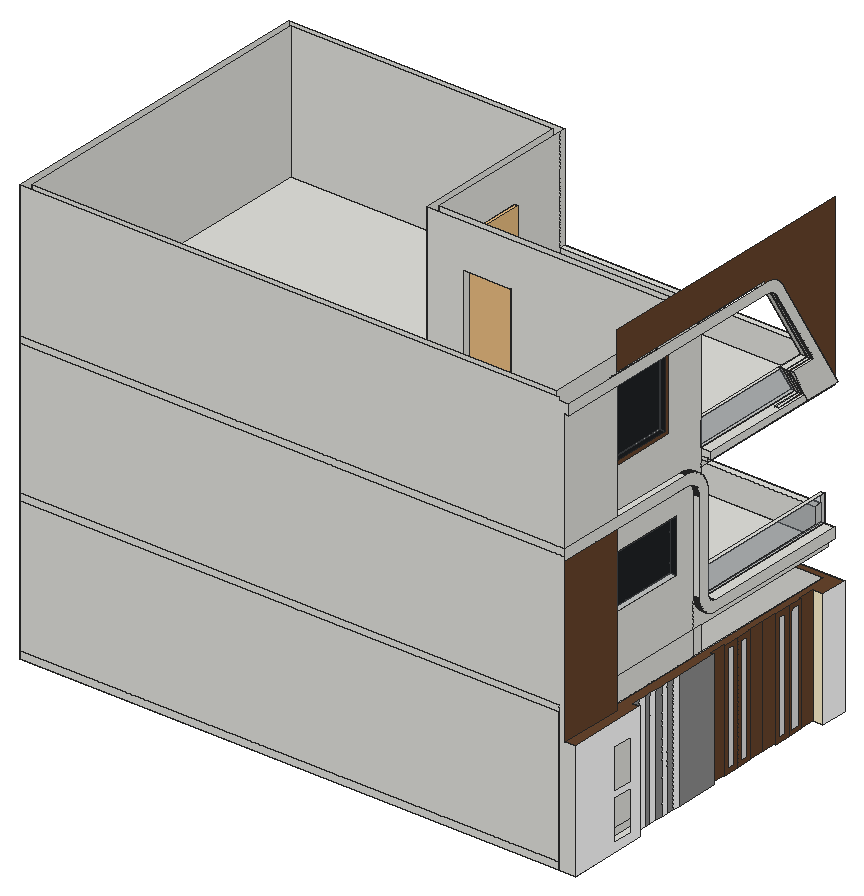
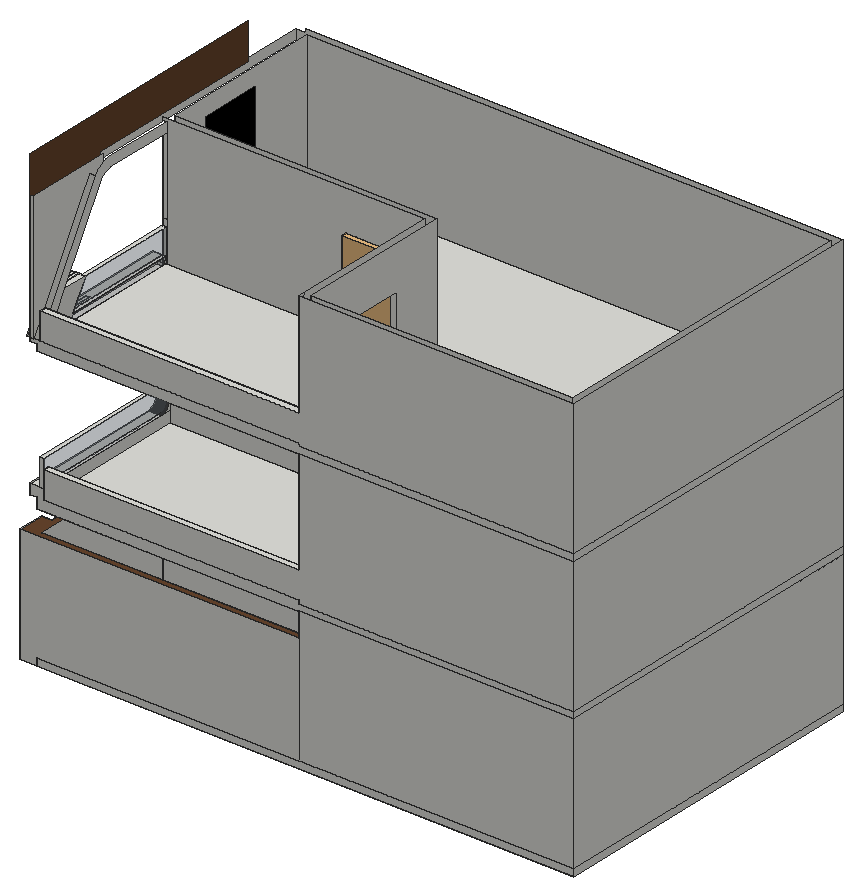
# SketchUp Ruby script. Lengths in inches.
U = 1.inch
M = Sketchup.active_model
def pt(a) = Geom::Point3d.new(a.map { |v| v * U })
def face(e, loops, mat)
  f = e.add_face(loops[0].map { |a| pt(a) })
  loops[1..].each { |l| e.add_face(l.map { |a| pt(a) }).erase! }
  f.material = f.back_material = mat if mat
  f
end
# faces: each face lists its corners as indices into pts; further lists are holes
def faces(e, pts, list, mat = nil) = list.each { |f| face(e, (f[0].is_a?(Array) ? f : [f]).map { |l| l.map { |i| pts[i] } }, mat) }
# xy, xz, yz: faces in a plane at the given z, y or x. An outline is a flat list of corners, or four numbers for a rectangle; further outlines are holes
def ring(l) = l.size == 4 ? [[l[0], l[1]], [l[2], l[1]], [l[2], l[3]], [l[0], l[3]]] : l.each_slice(2).to_a
def flat(e, list, mat, &to3) = list.each { |f| face(e, (f[0].is_a?(Array) ? f : [f]).map { |l| ring(l).map { |u, v| to3.(u, v) } }, mat) }
def xy(e, z, list, mat = nil) = flat(e, list, mat) { |x, y| [x, y, z] }
def xz(e, y, list, mat = nil) = flat(e, list, mat) { |x, z| [x, y, z] }
def yz(e, x, list, mat = nil) = flat(e, list, mat) { |y, z| [x, y, z] }
def lines(e, pts, list) = list.each { |a, b| e.add_line(pt(pts[a]), pt(pts[b])) }
# prism: a flat outline (further loops are holes) pulled along v
def prism(e, loops, v, mat = nil)
  f = face(e, loops, mat); d = Geom::Vector3d.new(v.map { |x| x * U })
  f.pushpull(f.normal.samedirection?(d) ? d.length : -d.length)
end
def box(e, o, s, mat = nil) = prism(e, [[o, [o[0] + s[0], o[1], o[2]], [o[0] + s[0], o[1] + s[1], o[2]], [o[0], o[1] + s[1], o[2]]]], [0, 0, s[2]], mat)
def at(x, y, z, deg = 0) = Geom::Transformation.translation(pt([x, y, z])) * Geom::Transformation.rotation(ORIGIN, Z_AXIS, deg.degrees)
def axes(o, x, y, z) = Geom::Transformation.new([*x, 0, *y, 0, *z, 0, *pt(o).to_a, 1])
def part(name) = M.definitions.add(name)
# library, detail: a bought-in or finely detailed component or shape, given as its bounding box
def library(name, o, s) = part(name).tap { |d| box(d.entities, o, s) }
def detail(e, o, s) = box(e.add_group.entities, o, s)
def put(e, d, t, mat = nil) = e.add_instance(d, t).tap { |i| i.material = mat if mat }
def group(e, t, mat = nil) = e.add_group.tap { |g| g.transformation = t; g.material = mat if mat }.entities
root = M.entities
M.materials.add("D01_Frost_White").color = [255, 242, 206]
M.materials.add("Glass_Basic_01").color = [130, 139, 150]
M.materials["Glass_Basic_01"].alpha = 0.25
M.materials.add("M00_Soft_Cloud").color = [255, 255, 255]
M.materials.add("M01_Silver_Fog").color = [224, 224, 224]
M.materials.add("M04_Stone_Frost").color = [142, 142, 142]
M.materials.add("M09_Shadow_Night").color = [0, 0, 0]
M.materials.add("Wood_Veneer_15_1K").color = [103, 69, 45]
c1 = library("porta+4",[0.2,-5.42,1.33],[46.55,4.72,83.21])
c2 = library("mesh-166",[-1553.69,-2604.3125,-42.18],[1702.88,1401.6,88.28])
c3 = part("Group17")
put(c3.entities,c2,at(294.66,859.51,3.5))
xy(root,-6,[[0,0,480,300],[480,0,480,300,495,300,495,276,486,276,486,261.75,487,261.75,487,233.25,486,233.25,486,204.75,487,204.75,487,176.25,486,176.25,486,162,489,162,489,72,495,72,495,0]])
xy(root,0,[[9,9,369,153],[375,9,471,153],[9,159,240,291],[246,159,471,291],[471,159,480,159,480,294,246,294,246,291,471,291],
  [246,294,480,300]])
xy(root,3,[[273,153,315,159]])
xy(root,39,[[240,198,246,240]])
xy(root,81,[[273,153,315,159],[240,198,246,240]])
xy(root,98.18,[[486,0,495,0,495,72,489,72,489,162,486,162,486,176.25,487,176.25,487,204.75,486,204.75,486,233.25,487,233.25,487,261.75,486,261.75,486,276,495,276,495,300,246,300,246,294,480,294,480,57,486,57]],"Wood_Veneer_15_1K")
xy(root,120,[[0,0,480,0,480,159,471,159,471,9,0,9],[0,9,9,300],[9,9,369,153],[369,9,375,159],[375,9,471,153],
  [9,153,369,153,369,159,246,159,246,300,240,300,240,159,9,159],[375,153,471,159],[9,159,240,291],[246,159,480,291],[9,291,240,300],
  [246,291,480,300]])
xy(root,126,[[6,6,474,6,474,153,240,153,240,294,6,294]])
xy(root,129,[[273,153,315,159],[246,159,474,294],[480,168,486,300],[246,294,474,300]])
xy(root,138,[[474,159,477,168],[474,168,477,300],[477,168,486,300]])
xy(root,153,[[246,294,474,300]])
xy(root,162,[[474,159,477,300]])
xy(root,165,[[240,198,246,240]])
xy(root,171,[[474,60,480,132]])
xy(root,207,[[273,153,315,159],[240,198,246,240]])
xy(root,219,[[474,60,480,108],[474,108,480,132]])
xy(root,243,[[480,57,486,135]])
xy(root,246,[[0,6,6,300],[6,6,6,294,240,294,240,153,474,153,474,6],[240,153,474,153,474,159,246,159,246,300,240,300],[246,159,480,300],[6,294,240,300]])
xy(root,252,[[6,6,474,6,474,153,240,153,240,294,6,294],[480,57,486,135],[480,159,486,300]])
xy(root,255,[[273,153,315,159],[246,159,477,294],[486,159,489,269.77],[483,237.63,486,269.77],[477,269.77,483,291],
  [483,269.77,486,291],[486,269.77,489,291],[477,291,483,300],[483,291,486,300],[486,291,489,300]])
xy(root,261,[[477,159,480,263.46],[480,159,489,159,489,263.46,486,263.46,486,237.63,483,237.63,483,263.46,480,263.46],[483,237.63,486,263.46]])
xy(root,279,[[246,294,477,300]])
xy(root,285,[[477,159,480,249.31],[477,249.31,483,273.31],[483,249.31,486,273.31],[486,249.31,489,273.31]])
xy(root,291,[[240,198,246,240]])
xy(root,291,[[474,63,480,120]],"M09_Shadow_Night")
xy(root,333,[[273,153,315,159],[240,198,246,240]])
xz(root,0,[[0,-6,480,0],[480,-6,495,-6,495,98.18,486,98.18,486,246,0,246,0,126,480,126],[0,0,480,120],[0,120,480,126],[0,246,486,252],
  [0,252,486,252,486,360,489,360,489,368.99,486,368.99,486,369,480,369,480,372,0,372]])
xz(root,6,[[6,126,474,246],[6,252,474,372]])
xz(root,9,[[9,0,369,120],[375,0,471,120]])
xz(root,57,[[480,98.18,486,243],[480,252,486,360]])
xz(root,60,[[474,171,480,219]])
xz(root,63,[[474,291,480,357]],"M09_Shadow_Night")
xz(root,72,[[489,-6,495,98.18]],"Wood_Veneer_15_1K")
xz(root,120,[[474,291,480,357]],"M09_Shadow_Night")
xz(root,132,[[474,171,480,219]],"M09_Shadow_Night")
xz(root,150,[[480,147,486,228]])
xz(root,153,[[[9,0,369,120],[273,3,315,81]],[375,0,471,120],[[240,126,474,246],[273,129,315,207]],[[240,252,474,372],[273,255,315,333]]])
xz(root,159,[[9,0,240,120],[246,0,246,120,480,120,480,0,318,0,318,84,270,84,270,0],[[270,0,318,84],[273,3,315,81]],[246,126,270,129],[270,126,318,129],
  [246,129,246,246,480,246,480,228,486,228,486,147,477,147,477,162,474,162,474,129,318,129,318,210,270,210,270,129],[270,129,270,210,318,210,318,129,315,129,315,207,273,207,273,129],[474,138,477,147],[474,147,477,162],[480,252,486,255],
  [246,255,246,372,480,372,480,369,477,369,477,255,318,255,318,336,270,336,270,255],[270,255,270,336,318,336,318,255,315,255,315,333,273,333,273,255],[477,255,480,261],[480,255,489,261],[477,261,480,285],
  [477,285,480,291],[477,291,480,360]])
xz(root,162,[[486,-6,489,98.18]],"Wood_Veneer_15_1K")
xz(root,176.25,[[486,-6,487,98.18]],"Wood_Veneer_15_1K")
xz(root,198,[[240,39,246,81],[240,165,246,207],[240,291,246,333]])
xz(root,204.75,[[486,-6,487,98.18]],"Wood_Veneer_15_1K")
xz(root,233.25,[[486,-6,487,98.18]],"Wood_Veneer_15_1K")
xz(root,237.63,[[483,255,486,261]])
xz(root,240,[[240,39,246,81],[240,165,246,207],[240,291,246,333]])
xz(root,261.75,[[486,-6,487,98.18]],"Wood_Veneer_15_1K")
xz(root,276,[[486,-6,495,98.18]],"D01_Frost_White")
xz(root,291,[[9,0,240,120]])
xz(root,294,[[246,0,480,98.18],[6,126,240,246],[246,129,474,153],[6,252,240,372],[246,255,477,279]])
xz(root,300,[[0,-6,480,0],[480,-6,480,0,246,0,246,98.18,495,98.18,495,-6],[0,0,246,120],[0,120,0,126,246,126,246,129,474,129,474,138,486,138,486,129,480,129,480,120],[0,126,0,246,246,246,246,153,474,153,474,129,246,129,246,126],
  [474,138,477,162],[0,246,0,252,246,252,246,255,486,255,486,252,480,252,480,246],[0,252,0,372,246,372,246,279,477,279,477,255,246,255,246,252],[483,255,486,369]])
yz(root,0,[[0,-6,300,0],[0,0,300,120],[0,120,300,126],[0,126,300,246],[0,246,300,252],
  [0,252,300,372]])
yz(root,6,[[6,126,294,246],[6,252,294,372]])
yz(root,9,[[9,0,153,120],[153,0,159,120],[159,0,291,120]])
yz(root,240,[[[159,0,291,120],[198,39,240,81]],[[153,126,294,246],[198,165,240,207]],[[153,252,294,372],[198,291,240,333]]])
yz(root,246,[[[159,0,294,0,294,98.18,300,98.18,300,120,159,120],[195,36,243,84]],[[195,36,243,84],[198,39,240,81]],[159,126,300,129],[[159,129,294,246],[195,162,243,210]],[294,153,300,246],
  [[195,162,243,210],[198,165,240,207]],[[159,255,294,372],[195,288,243,336]],[294,279,300,372],[[195,288,243,336],[198,291,240,333]]])
yz(root,273,[[153,3,159,81],[153,129,159,207],[153,255,159,333]])
yz(root,315,[[153,3,159,81],[153,129,159,207],[153,255,159,333]])
yz(root,369,[[9,0,153,120]])
yz(root,375,[[9,0,153,120]])
yz(root,471,[[9,0,153,120]])
yz(root,474,[[[6,126,153,246],[60,171,132,219]],[159,129,294,138],[294,129,300,138],[159,138,159,147,159.01,146.72,159.03,146.4375,159.06,146.16,159.14,145.6,159.26,145.06,159.33,144.78,159.41,144.51,159.49,144.25,159.59,143.98,159.69,143.72,159.8,143.46,159.92,143.21,160.18,142.71,160.32,142.47,160.47,142.23,160.79,141.77,160.96,141.54,161.14,141.33,161.32,141.11,161.51,140.91,161.7,140.7,161.91,140.51,162.11,140.32,162.33,140.14,162.54,139.96,162.77,139.79,163.23,139.47,163.47,139.32,163.71,139.18,164.21,138.92,164.46,138.8,164.72,138.69,164.98,138.59,165.25,138.49,165.51,138.41,165.78,138.33,166.06,138.26,166.6,138.14,167.16,138.06,167.4375,138.03,167.72,138.01,168,138],[294,138,300,153],
  [[6,252,153,372],[63,291,120,357]]])
yz(root,474,[[168,138,167.72,138.01,167.4375,138.03,167.16,138.06,166.6,138.14,166.06,138.26,165.78,138.33,165.51,138.41,165.25,138.49,164.98,138.59,164.72,138.69,164.46,138.8,164.21,138.92,163.71,139.18,163.47,139.32,163.23,139.47,162.77,139.79,162.54,139.96,162.33,140.14,162.11,140.32,161.91,140.51,161.7,140.7,161.51,140.91,161.32,141.11,161.14,141.33,160.96,141.54,160.79,141.77,160.47,142.23,160.32,142.47,160.18,142.71,159.92,143.21,159.8,143.46,159.69,143.72,159.59,143.98,159.49,144.25,159.41,144.51,159.33,144.78,159.26,145.06,159.14,145.6,159.06,146.16,159.03,146.4375,159.01,146.72,159,147,159,162,300,162,300,153,294,153,294,138]],"Glass_Basic_01")
yz(root,474,[[60,171,132,219],[63,291,120,357]],"M09_Shadow_Night")
yz(root,477,[[291,255,273.31,285,232.23,354.64,231.91,355.06,231.57,355.46,231.39,355.66,231.03,356.04,230.46,356.58,230.26,356.76,230.06,356.92,229.85,357.09,229.43,357.41,229.22,357.5625,229,357.71,228.78,357.86,228.56,358,228.33,358.14,228.11,358.27,227.875,358.4,227.64,358.52,227.41,358.64,226.93,358.86,226.6875,358.96,226.44,359.06,226.2,359.16,225.95,359.25,225.7,359.33,225.45,359.42,225.2,359.49,224.94,359.5625,224.6875,359.625,224.43,359.6875,224.17,359.74,223.92,359.79,223.66,359.84,223.4,359.88,223.13,359.91,222.61,359.97,222.35,359.99,222.15,360,159,360,159,369,222.39,369,222.39,368.92,222.53,368.91,222.97,368.89,223.41,368.85,223.84,368.81,224.72,368.69,225.58,368.53,226.44,368.33,226.87,368.21,227.29,368.09,227.71,367.96,228.125,367.82,228.54,367.67,228.95,367.51,229.08,367.45,229.36,367.34,229.76,367.16,230.16,366.97,230.55,366.78,231.33,366.36,231.71,366.14,232.08,365.9,232.45,365.67,232.81,365.42,233.53,364.9,233.875,364.63,234.21,364.35,234.55,364.0625,234.875,363.77,235.2,363.47,235.82,362.85,236.12,362.52,236.7,361.86,236.98,361.52,237.25,361.17,237.51,360.82,237.76,360.46,238.01,360.09,238.07,360,238.14,359.9,294,265.17,294,255],[267,255,263.46,261,249.31,285,273.31,285,291,255],[294,255,294,265.17,300,255],[300,255,300,279,294,279,294,265.17]])
yz(root,477,[[159,138,300,162],[159,255,159,261,162.54,255],[162.54,255,159,261,263.46,261,267,255],[159,261,159,285,249.31,285,263.46,261]],"Glass_Basic_01")
yz(root,480,[[0,-6,300,0],[0,0,159,0,159,98.18,57,98.18,57,120,0,120],[159,0,294,98.18],[57,98.18,150,120],[150,98.18,159,120],
  [[57,120,150,120,150,228,149.98,228.47,149.95,228.9375,149.91,229.4,149.85,229.87,149.77,230.33,149.68,230.79,149.58,231.25,149.46,231.7,149.33,232.15,149.19,232.6,149.03,233.04,148.86,233.47,148.68,233.9,148.48,234.33,148.27,234.75,148.05,235.16,147.8125,235.57,147.57,235.96,147.31,236.35,147.04,236.74,146.75,237.11,146.46,237.47,146.15,237.83,145.84,238.18,145.18,238.84,144.83,239.15,144.47,239.46,144.11,239.75,143.74,240.04,143.35,240.31,142.96,240.57,142.57,240.8125,142.16,241.05,141.75,241.27,141.33,241.48,140.9,241.68,140.47,241.86,140.04,242.03,139.6,242.19,139.15,242.33,138.7,242.46,138.25,242.58,137.79,242.68,137.33,242.77,136.87,242.85,136.4,242.91,135.9375,242.95,135.47,242.98,135,243,57,243],[60,171,132,219]],[150,120,300,120,300,129,168,129,167.4375,129.01,166.875,129.05,166.3125,129.1,165.75,129.16,165.19,129.25,164.64,129.35,164.09,129.47,163.54,129.6,163,129.75,162.46,129.92,161.93,130.11,161.4,130.3125,160.88,130.53,160.37,130.76,159.86,131.02,159.37,131.28,158.875,131.5625,158.4,131.86,157.93,132.17,157.47,132.49,157.02,132.83,156.58,133.1875,156.15,133.55,155.73,133.93,154.93,134.73,154.55,135.15,154.1875,135.58,153.83,136.02,153.49,136.47,153.17,136.93,152.86,137.4,152.5625,137.875,152.28,138.37,152.02,138.86,151.76,139.37,151.53,139.88,151.3125,140.4,151.11,140.93,150.92,141.46,150.75,142,150.6,142.54,150.47,143.09,150.35,143.64,150.25,144.19,150.16,144.75,150.1,145.3125,150.05,145.875,150.01,146.4375,150,147],[159,228,159,360,123,360,123,288,60,288,60,360,57,360,57,252,135,252,135.75,251.99,136.51,251.96,137.26,251.9,138.01,251.82,138.76,251.72,139.5,251.59,140.24,251.44,140.98,251.27,141.71,251.07,142.43,250.85,143.14,250.61,143.85,250.34,144.55,250.06,145.24,249.75,145.92,249.42,146.58,249.0625,147.24,248.69,147.88,248.3,148.52,247.88,149.13,247.45,149.74,247,150,246.79,150.33,246.53,150.9,246.04,151.46,245.53,152,245,152.53,244.46,153.04,243.9,153.53,243.33,154,242.74,154.45,242.13,154.88,241.52,155.3,240.88,155.69,240.24,156.0625,239.58,156.42,238.92,156.75,238.24,157.06,237.55,157.34,236.85,157.61,236.14,157.85,235.43,158.07,234.71,158.27,233.98,158.44,233.24,158.59,232.5,158.72,231.76,158.82,231.01,158.9,230.26,158.96,229.51,158.99,228.75],[159,246,300,252]])
yz(root,480,[[60,171,132,219],[159,261,263.46,261,249.31,285,159,285],[63,291,120,357]],"Glass_Basic_01")
yz(root,480,[[[60,288,123,360],[63,291,120,357]]],"Wood_Veneer_15_1K")
yz(root,483,[[237.63,255,237.63,261,263.46,261,249.31,285,273.31,285,237.63,345.49,232.23,354.64,232.09,354.83,231.95,355.01,231.8,355.18,231.65,355.36,231.49,355.53,231.34,355.7,231.18,355.87,231.01,356.03,230.85,356.2,230.68,356.36,230.51,356.51,230.33,356.67,230.16,356.82,229.98,356.96,229.8,357.11,229.62,357.25,229.43,357.39,228.86,357.78,228.66,357.91,228.47,358.03,228.27,358.15,228.07,358.26,227.86,358.375,227.66,358.48,227.45,358.59,227.03,358.79,226.61,358.97,226.4,359.0625,226.18,359.14,225.74,359.3,225.08,359.51,224.86,359.57,224.63,359.625,224.41,359.68,224.18,359.73,223.95,359.77,223.73,359.82,223.5,359.86,222.81,359.95,222.58,359.97,222.39,359.99,222.39,369,300,369,300,255]])
yz(root,486,[[168,129,300,129,300,138,168,138,167.72,138.01,167.4375,138.03,167.16,138.06,166.6,138.14,166.06,138.26,165.78,138.33,165.51,138.41,165.25,138.49,164.98,138.59,164.72,138.69,164.46,138.8,164.21,138.92,163.71,139.18,163.47,139.32,163.23,139.47,162.77,139.79,162.54,139.96,162.33,140.14,162.11,140.32,161.91,140.51,161.7,140.7,161.51,140.91,161.32,141.11,161.14,141.33,160.96,141.54,160.79,141.77,160.47,142.23,160.32,142.47,160.18,142.71,159.92,143.21,159.8,143.46,159.69,143.72,159.59,143.98,159.49,144.25,159.41,144.51,159.33,144.78,159.26,145.06,159.14,145.6,159.06,146.16,159.03,146.4375,159.01,146.72,159,147,159,228,158.99,228.75,158.96,229.51,158.9,230.26,158.82,231.01,158.72,231.76,158.59,232.5,158.44,233.24,158.27,233.98,158.07,234.71,157.85,235.43,157.61,236.14,157.34,236.85,157.06,237.55,156.75,238.24,156.42,238.92,156.0625,239.58,155.69,240.24,155.3,240.88,154.88,241.52,154.45,242.13,154,242.74,153.53,243.33,153.04,243.9,152.53,244.46,152,245,151.46,245.53,150.9,246.04,150.33,246.53,150,246.79,149.74,247,149.13,247.45,148.52,247.88,147.88,248.3,147.24,248.69,146.58,249.0625,145.92,249.42,145.24,249.75,144.55,250.06,143.85,250.34,143.14,250.61,142.43,250.85,141.71,251.07,140.98,251.27,140.24,251.44,139.5,251.59,138.76,251.72,138.01,251.82,137.26,251.9,136.51,251.96,135.75,251.99,135,252,0,252,0,243,135,243,135.47,242.98,135.9375,242.95,136.4,242.91,136.87,242.85,137.33,242.77,137.79,242.68,138.25,242.58,138.7,242.46,139.15,242.33,139.6,242.19,140.04,242.03,140.47,241.86,140.9,241.68,141.33,241.48,141.75,241.27,142.16,241.05,142.57,240.8125,142.96,240.57,143.35,240.31,143.74,240.04,144.11,239.75,144.47,239.46,144.83,239.15,145.18,238.84,145.84,238.18,146.15,237.83,146.46,237.47,146.75,237.11,147.04,236.74,147.31,236.35,147.57,235.96,147.8125,235.57,148.05,235.16,148.27,234.75,148.48,234.33,148.68,233.9,148.86,233.47,149.03,233.04,149.19,232.6,149.33,232.15,149.46,231.7,149.58,231.25,149.68,230.79,149.77,230.33,149.85,229.87,149.91,229.4,149.95,228.9375,149.98,228.47,150,228,150,147,150.01,146.4375,150.05,145.875,150.1,145.3125,150.16,144.75,150.25,144.19,150.35,143.64,150.47,143.09,150.6,142.54,150.75,142,150.92,141.46,151.11,140.93,151.3125,140.4,151.53,139.88,151.76,139.37,152.02,138.86,152.28,138.37,152.5625,137.875,152.86,137.4,153.17,136.93,153.49,136.47,153.83,136.02,154.1875,135.58,154.55,135.15,154.93,134.73,155.73,133.93,156.15,133.55,156.58,133.1875,157.02,132.83,157.47,132.49,157.93,132.17,158.4,131.86,158.875,131.5625,159.37,131.28,159.86,131.02,160.37,130.76,160.88,130.53,161.4,130.3125,161.93,130.11,162.46,129.92,163,129.75,163.54,129.6,164.09,129.47,164.64,129.35,165.19,129.25,165.75,129.16,166.3125,129.1,166.875,129.05,167.4375,129.01],[0,252,57,360],[159,252,300,255]])
yz(root,486,[[162,-6,176.25,98.18],[204.75,-6,219,98.18],[219,-6,233.25,98.18],[261.75,-6,276,98.18],[0,98.18,57,243],
  [237.63,255,300,255,300,402,57,402,57,369,222.39,369,222.39,359.99,222.58,359.97,222.81,359.95,223.5,359.86,223.73,359.82,223.95,359.77,224.18,359.73,224.41,359.68,224.63,359.625,224.86,359.57,225.08,359.51,225.74,359.3,226.18,359.14,226.4,359.0625,226.61,358.97,227.03,358.79,227.45,358.59,227.66,358.48,227.86,358.375,228.07,358.26,228.27,358.15,228.47,358.03,228.66,357.91,228.86,357.78,229.43,357.39,229.62,357.25,229.8,357.11,229.98,356.96,230.16,356.82,230.33,356.67,230.51,356.51,230.68,356.36,230.85,356.2,231.01,356.03,231.18,355.87,231.34,355.7,231.49,355.53,231.65,355.36,231.8,355.18,231.95,355.01,232.09,354.83,232.23,354.64,237.63,345.49,273.31,285,249.31,285,263.46,261,237.63,261]],"Wood_Veneer_15_1K")
yz(root,487,[[180.25,-2,186.5,94.18],[194.5,-2,200.75,94.18],[237.25,-2,243.5,94.18],[251.5,-2,257.75,94.18]],"M01_Silver_Fog")
yz(root,487,[[[176.25,-6,190.5,98.18],[180.25,-2,186.5,94.18]],[[190.5,-6,204.75,98.18],[194.5,-2,200.75,94.18]],[[233.25,-6,247.5,98.18],[237.25,-2,243.5,94.18]],[[247.5,-6,261.75,98.18],[251.5,-2,257.75,94.18]]],"Wood_Veneer_15_1K")
yz(root,489,[[267,255,300,255,238.91,358.58,238.14,359.9,238.01,360.09,237.76,360.46,237.51,360.82,237.25,361.17,236.98,361.52,236.7,361.86,236.12,362.52,235.82,362.85,235.2,363.47,234.875,363.77,234.55,364.0625,234.21,364.35,233.875,364.63,233.53,364.9,232.81,365.42,232.45,365.67,232.08,365.9,231.71,366.14,231.33,366.36,230.55,366.78,230.16,366.97,229.76,367.16,229.36,367.34,228.95,367.51,228.54,367.67,228.125,367.82,227.71,367.96,227.29,368.09,226.87,368.21,226.44,368.33,225.58,368.53,224.72,368.69,223.84,368.81,223.41,368.85,222.97,368.89,222.53,368.91,222.39,368.92,222.39,368.97,214.74,369,57,369,57,368.99,0,368.99,0,360,220.77,360,221.29,360.02,221.56,360.02,222.08,360,222.15,360,222.35,359.99,222.61,359.97,223.13,359.91,223.4,359.88,223.66,359.84,223.92,359.79,224.17,359.74,224.43,359.6875,224.6875,359.625,224.94,359.5625,225.2,359.49,225.45,359.42,225.7,359.33,225.95,359.25,226.2,359.16,226.44,359.06,226.6875,358.96,226.93,358.86,227.41,358.64,227.64,358.52,227.875,358.4,228.11,358.27,228.33,358.14,228.56,358,228.78,357.86,229,357.71,229.22,357.5625,229.43,357.41,229.85,357.09,230.06,356.92,230.26,356.76,230.46,356.58,231.03,356.04,231.39,355.66,231.57,355.46,231.91,355.06,232.23,354.64,273.31,285,249.31,285,263.46,261],[159,255,267,255,263.46,261,159,261]])
yz(root,489,[[78.29,-6,84.57,98.18],[90.86,-6,97.14,98.18],[103.43,-6,109.72,98.18],[116,-6,122.29,98.18]],"M00_Soft_Cloud")
yz(root,489,[[72,-6,78.29,98.18],[84.57,-6,90.86,98.18],[97.14,-6,103.43,98.18],[109.72,-6,116,98.18],[122.29,-6,162,98.18]],"M04_Stone_Frost")
yz(root,495,[[[0,-6,72,98.18],[43.35,42.25,61.35,78.25],[43.35,1.43,61.35,37.43]],[276,-6,300,98.18]],"M00_Soft_Cloud")
p = [[480,166.3125,129.1],[480,166.875,129.05],[486,166.875,129.05],[486,166.3125,129.1],[480,167.4375,129.01],[486,167.4375,129.01],
  [480,168,129],[486,168,129],[480,165.75,129.16],[486,165.75,129.16],[480,164.64,129.35],[480,165.19,129.25],
  [486,165.19,129.25],[486,164.64,129.35],[480,164.09,129.47],[486,164.09,129.47],[480,163.54,129.6],[486,163.54,129.6],
  [480,163,129.75],[486,163,129.75],[480,162.46,129.92],[486,162.46,129.92],[480,161.93,130.11],[486,161.93,130.11],
  [480,161.4,130.3125],[486,161.4,130.3125],[480,160.88,130.53],[486,160.88,130.53],[480,160.37,130.76],[486,160.37,130.76],
  [480,159.86,131.02],[486,159.86,131.02],[480,159.37,131.28],[486,159.37,131.28],[480,158.875,131.5625],[486,158.875,131.5625],
  [480,158.4,131.86],[486,158.4,131.86],[480,157.93,132.17],[486,157.93,132.17],[480,157.47,132.49],[486,157.47,132.49],
  [480,157.02,132.83],[486,157.02,132.83],[480,156.58,133.1875],[486,156.58,133.1875],[480,156.15,133.55],[486,156.15,133.55],
  [480,155.73,133.93],[486,155.73,133.93],[480,155.33,134.33],[486,155.33,134.33],[480,154.93,134.73],[486,154.93,134.73],
  [480,154.55,135.15],[486,154.55,135.15],[480,154.1875,135.58],[486,154.1875,135.58],[480,153.83,136.02],[486,153.83,136.02],
  [480,153.49,136.47],[486,153.49,136.47],[480,153.17,136.93],[486,153.17,136.93],[480,152.86,137.4],[486,152.86,137.4],
  [480,152.5625,137.875],[486,152.5625,137.875],[480,152.28,138.37],[486,152.28,138.37],[474,167.16,138.06],[486,167.16,138.06],
  [486,167.4375,138.03],[474,167.4375,138.03],[486,167.72,138.01],[474,167.72,138.01],[486,168,138],[477,168,138],
  [474,168,138],[474,166.33,138.2],[486,166.33,138.2],[486,166.6,138.14],[474,166.6,138.14],[486,166.88,138.1],
  [474,166.88,138.1],[474,166.06,138.26],[486,166.06,138.26],[474,165.51,138.41],[486,165.51,138.41],[486,165.78,138.33],
  [474,165.78,138.33],[480,152.02,138.86],[486,152.02,138.86],[474,165.25,138.49],[486,165.25,138.49],[474,164.98,138.59],
  [486,164.98,138.59],[474,164.72,138.69],[486,164.72,138.69],[474,164.46,138.8],[486,164.46,138.8],[474,164.21,138.92],
  [486,164.21,138.92],[480,151.76,139.37],[486,151.76,139.37],[474,163.96,139.05],[486,163.96,139.05],[474,163.71,139.18],
  [486,163.71,139.18],[474,163.47,139.32],[486,163.47,139.32],[474,163.23,139.47],[486,163.23,139.47],[480,151.53,139.88],
  [486,151.53,139.88],[474,163,139.63],[486,163,139.63],[474,162.77,139.79],[486,162.77,139.79],[474,162.54,139.96],
  [486,162.54,139.96],[480,151.3125,140.4],[486,151.3125,140.4],[474,162.33,140.14],[486,162.33,140.14],[474,162.11,140.32],
  [486,162.11,140.32],[474,161.91,140.51],[486,161.91,140.51],[480,151.11,140.93],[486,151.11,140.93],[474,161.7,140.7],
  [486,161.7,140.7],[474,161.51,140.91],[486,161.51,140.91],[480,150.92,141.46],[486,150.92,141.46],[474,161.32,141.11],
  [486,161.32,141.11],[474,161.14,141.33],[486,161.14,141.33],[474,160.96,141.54],[486,160.96,141.54],[480,150.75,142],
  [486,150.75,142],[474,160.79,141.77],[486,160.79,141.77],[474,160.63,142],[486,160.63,142],[480,150.6,142.54],
  [486,150.6,142.54],[474,160.47,142.23],[486,160.47,142.23],[474,160.32,142.47],[486,160.32,142.47],[480,150.47,143.09],
  [486,150.47,143.09],[474,160.18,142.71],[486,160.18,142.71],[474,160.05,142.96],[486,160.05,142.96],[474,159.92,143.21],
  [486,159.92,143.21],[480,150.35,143.64],[486,150.35,143.64],[474,159.8,143.46],[486,159.8,143.46],[474,159.69,143.72],
  [486,159.69,143.72],[480,150.25,144.19],[486,150.25,144.19],[474,159.59,143.98],[486,159.59,143.98],[474,159.49,144.25],
  [486,159.49,144.25],[480,150.16,144.75],[486,150.16,144.75],[474,159.41,144.51],[486,159.41,144.51],[474,159.33,144.78],
  [486,159.33,144.78],[480,150.1,145.3125],[486,150.1,145.3125],[474,159.26,145.06],[486,159.26,145.06],[474,159.2,145.33],
  [486,159.2,145.33],[480,150.05,145.875],[486,150.05,145.875],[474,159.14,145.6],[486,159.14,145.6],[474,159.1,145.88],
  [486,159.1,145.88],[480,150.01,146.4375],[486,150.01,146.4375],[474,159.06,146.16],[486,159.06,146.16],[474,159.03,146.4375],
  [486,159.03,146.4375],[480,150,147],[486,150,147],[474,159.01,146.72],[486,159.01,146.72],[477,159,147],
  [486,159,147],[474,159,147],[480,149.98,228.47],[480,150,228],[486,150,228],[486,149.98,228.47],
  [480,159,228],[480,158.99,228.75],[486,158.99,228.75],[486,159,228],[480,149.95,228.9375],[486,149.95,228.9375],
  [480,158.96,229.51],[486,158.96,229.51],[480,149.91,229.4],[486,149.91,229.4],[480,149.85,229.87],[486,149.85,229.87],
  [480,158.9,230.26],[486,158.9,230.26],[480,149.77,230.33],[486,149.77,230.33],[480,149.68,230.79],[486,149.68,230.79],
  [480,158.82,231.01],[486,158.82,231.01],[480,149.58,231.25],[486,149.58,231.25],[480,158.72,231.76],[486,158.72,231.76],
  [480,149.46,231.7],[486,149.46,231.7],[480,149.33,232.15],[486,149.33,232.15],[480,158.59,232.5],[486,158.59,232.5],
  [480,149.19,232.6],[486,149.19,232.6],[480,158.44,233.24],[486,158.44,233.24],[480,149.03,233.04],[486,149.03,233.04],
  [480,148.86,233.47],[486,148.86,233.47],[480,158.27,233.98],[486,158.27,233.98],[480,148.68,233.9],[486,148.68,233.9],
  [480,148.48,234.33],[486,148.48,234.33],[480,158.07,234.71],[486,158.07,234.71],[480,148.27,234.75],[486,148.27,234.75],
  [480,148.05,235.16],[486,148.05,235.16],[480,157.85,235.43],[486,157.85,235.43],[480,147.8125,235.57],[486,147.8125,235.57],
  [480,157.61,236.14],[486,157.61,236.14],[480,147.57,235.96],[486,147.57,235.96],[480,147.31,236.35],[486,147.31,236.35],
  [480,157.34,236.85],[486,157.34,236.85],[480,147.04,236.74],[486,147.04,236.74],[480,146.75,237.11],[486,146.75,237.11],
  [480,157.06,237.55],[486,157.06,237.55],[480,146.46,237.47],[486,146.46,237.47],[480,146.15,237.83],[486,146.15,237.83],
  [480,156.75,238.24],[486,156.75,238.24],[480,145.84,238.18],[486,145.84,238.18],[480,145.51,238.51],[486,145.51,238.51],
  [480,156.42,238.92],[486,156.42,238.92],[480,145.18,238.84],[486,145.18,238.84],[480,144.83,239.15],[486,144.83,239.15],
  [480,156.0625,239.58],[486,156.0625,239.58],[480,144.47,239.46],[486,144.47,239.46],[480,144.11,239.75],[486,144.11,239.75],
  [480,155.69,240.24],[486,155.69,240.24],[480,143.74,240.04],[486,143.74,240.04],[480,143.35,240.31],[486,143.35,240.31],
  [480,155.3,240.88],[486,155.3,240.88],[480,142.96,240.57],[486,142.96,240.57],[480,142.57,240.8125],[486,142.57,240.8125],
  [480,142.16,241.05],[486,142.16,241.05],[480,154.88,241.52],[486,154.88,241.52],[480,141.75,241.27],[486,141.75,241.27],
  [480,141.33,241.48],[486,141.33,241.48],[480,140.9,241.68],[486,140.9,241.68],[480,154.45,242.13],[486,154.45,242.13],
  [480,140.47,241.86],[486,140.47,241.86],[480,140.04,242.03],[486,140.04,242.03],[480,139.6,242.19],[486,139.6,242.19],
  [480,154,242.74],[486,154,242.74],[480,139.15,242.33],[486,139.15,242.33],[480,138.7,242.46],[486,138.7,242.46],
  [480,138.25,242.58],[486,138.25,242.58],[480,137.79,242.68],[486,137.79,242.68],[480,137.33,242.77],[486,137.33,242.77],
  [480,153.53,243.33],[486,153.53,243.33],[480,136.4,242.91],[480,136.87,242.85],[486,136.87,242.85],[486,136.4,242.91],
  [480,135.9375,242.95],[486,135.9375,242.95],[480,135,243],[480,135.47,242.98],[486,135.47,242.98],[486,135,243],
  [480,153.04,243.9],[486,153.04,243.9],[480,152.53,244.46],[486,152.53,244.46],[480,152,245],[486,152,245],
  [480,151.46,245.53],[486,151.46,245.53],[480,150.9,246.04],[486,150.9,246.04],[480,150.33,246.53],[486,150.33,246.53],
  [480,150,246.79],[486,150,246.79],[480,149.74,247],[486,149.74,247],[480,149.13,247.45],[486,149.13,247.45],
  [480,148.52,247.88],[486,148.52,247.88],[480,147.88,248.3],[486,147.88,248.3],[480,147.24,248.69],[486,147.24,248.69],
  [480,146.58,249.0625],[486,146.58,249.0625],[480,145.92,249.42],[486,145.92,249.42],[480,145.24,249.75],[486,145.24,249.75],
  [480,144.55,250.06],[486,144.55,250.06],[480,143.85,250.34],[486,143.85,250.34],[480,143.14,250.61],[486,143.14,250.61],
  [480,142.43,250.85],[486,142.43,250.85],[480,141.71,251.07],[486,141.71,251.07],[480,140.98,251.27],[486,140.98,251.27],
  [480,140.24,251.44],[486,140.24,251.44],[480,139.5,251.59],[486,139.5,251.59],[480,138.76,251.72],[486,138.76,251.72],
  [480,138.01,251.82],[486,138.01,251.82],[480,137.26,251.9],[486,137.26,251.9],[480,136.51,251.96],[486,136.51,251.96],
  [480,135.75,251.99],[480,135,252],[486,135,252],[486,135.75,251.99],[489,300,255],[486,300,255],
  [483,300,255],[477,300,255],[477,294,265.17],[477,238.14,359.9],[486,238.14,359.9],[489,238.14,359.9],
  [489,238.91,358.58],[477,249.31,285],[477,263.46,261],[480,263.46,261],[480,249.31,285],[483,263.46,261],
  [483,249.31,285],[486,263.46,261],[486,249.31,285],[489,249.31,285],[489,263.46,261],[483,273.31,285],
  [483,237.63,345.49],[483,232.23,354.64],[477,232.23,354.64],[477,273.31,285],[489,232.23,354.64],[486,232.23,354.64],
  [486,237.63,345.49],[486,273.31,285],[489,273.31,285],[480,45,243],[480,45,252],[477,159,138],
  [480,159,138]]
faces(root,p,[[0,1,2,3],[1,4,5,2],[4,6,7,5],[8,0,3,9],[10,11,12,13],[11,8,9,12],[14,10,13,15],[16,14,15,17],
  [18,16,17,19],[20,18,19,21],[22,20,21,23],[24,22,23,25],[26,24,25,27],[28,26,27,29],[30,28,29,31],[32,30,31,33],
  [34,32,33,35],[36,34,35,37],[38,36,37,39],[40,38,39,41],[42,40,41,43],[44,42,43,45],[46,44,45,47],[48,46,47,49],
  [50,48,49,51],[52,50,51,53],[54,52,53,55],[56,54,55,57],[58,56,57,59],[60,58,59,61],[62,60,61,63],[64,62,63,65],
  [66,64,65,67],[68,66,67,69],[70,71,72,73],[73,72,74,75],[75,74,76,77,78],[79,80,81,82],[82,81,83,84],[84,83,71,70],
  [85,86,80,79],[87,88,89,90],[90,89,86,85],[91,68,69,92],[93,94,88,87],[95,96,94,93],[97,98,96,95],[99,100,98,97],
  [101,102,100,99],[103,91,92,104],[105,106,102,101],[107,108,106,105],[109,110,108,107],[111,112,110,109],[113,103,104,114],[115,116,112,111],
  [117,118,116,115],[119,120,118,117],[121,113,114,122],[123,124,120,119],[125,126,124,123],[127,128,126,125],[129,121,122,130],[131,132,128,127],
  [133,134,132,131],[135,129,130,136],[137,138,134,133],[139,140,138,137],[141,142,140,139],[143,135,136,144],[145,146,142,141],[147,148,146,145],
  [149,143,144,150],[151,152,148,147],[153,154,152,151],[155,149,150,156],[157,158,154,153],[159,160,158,157],[161,162,160,159],[163,155,156,164],
  [165,166,162,161],[167,168,166,165],[169,163,164,170],[171,172,168,167],[173,174,172,171],[175,169,170,176],[177,178,174,173],[179,180,178,177],
  [181,175,176,182],[183,184,180,179],[185,186,184,183],[187,181,182,188],[189,190,186,185],[191,192,190,189],[193,187,188,194],[195,196,192,191],
  [197,198,196,195],[199,193,194,200],[201,202,198,197],[203,204,202,201,205],[206,207,208,209],[210,211,212,213],[214,206,209,215],[211,216,217,212],
  [218,214,215,219],[220,218,219,221],[216,222,223,217],[224,220,221,225],[226,224,225,227],[222,228,229,223],[230,226,227,231],[228,232,233,229],
  [234,230,231,235],[236,234,235,237],[232,238,239,233],[240,236,237,241],[238,242,243,239],[244,240,241,245],[246,244,245,247],[242,248,249,243],
  [250,246,247,251],[252,250,251,253],[248,254,255,249],[256,252,253,257],[258,256,257,259],[254,260,261,255],[262,258,259,263],[260,264,265,261],
  [266,262,263,267],[268,266,267,269],[264,270,271,265],[272,268,269,273],[274,272,273,275],[270,276,277,271],[278,274,275,279],[280,278,279,281],
  [276,282,283,277],[284,280,281,285],[286,284,285,287],[282,288,289,283],[290,286,287,291],[292,290,291,293],[288,294,295,289],[296,292,293,297],
  [298,296,297,299],[294,300,301,295],[302,298,299,303],[304,302,303,305],[300,306,307,301],[308,304,305,309],[310,308,309,311],[312,310,311,313],
  [306,314,315,307],[316,312,313,317],[318,316,317,319],[320,318,319,321],[314,322,323,315],[324,320,321,325],[326,324,325,327],[328,326,327,329],
  [322,330,331,323],[332,328,329,333],[334,332,333,335],[336,334,335,337],[338,336,337,339],[340,338,339,341],[330,342,343,331],[344,345,346,347],
  [345,340,341,346],[348,344,347,349],[350,351,352,353],[351,348,349,352],[342,354,355,343],[354,356,357,355],[356,358,359,357],[358,360,361,359],
  [360,362,363,361],[362,364,365,363],[364,366,367,365],[366,368,369,367],[368,370,371,369],[370,372,373,371],[372,374,375,373],[374,376,377,375],
  [376,378,379,377],[378,380,381,379],[380,382,383,381],[382,384,385,383],[384,386,387,385],[386,388,389,387],[388,390,391,389],[390,392,393,391],
  [392,394,395,393],[394,396,397,395],[396,398,399,397],[398,400,401,399],[400,402,403,401],[402,404,405,403],[404,406,407,405],[408,409,410,411],
  [406,408,411,407],[412,413,414,415,416,417,418,419,420],[421,422,423,424],[423,425,426,424],[427,428,426,425],[429,428,427,430],[431,432,433,434,435],[436,437,438,439,440],
  [431,439,438,432],[438,437,433,432]])
lines(root,p,[[441,442],[443,444]])
put(root,c1,at(269.8,164.42,-0.54))
put(root,c3,axes([247.52,230.5,95.89],[0,0.02817,0],[0,0,0.03465],[0.03937,0,0]))
put(root,c1,at(269.8,164.42,125.46))
put(root,c3,axes([247.52,230.5,222.45],[0,0.02817,0],[0,0,0.03465],[0.03937,0,0]))
put(root,c1,at(269.8,164.42,251.46))
put(root,c3,axes([247.52,230.5,348.45],[0,0.02817,0],[0,0,0.03465],[0.03937,0,0]))
